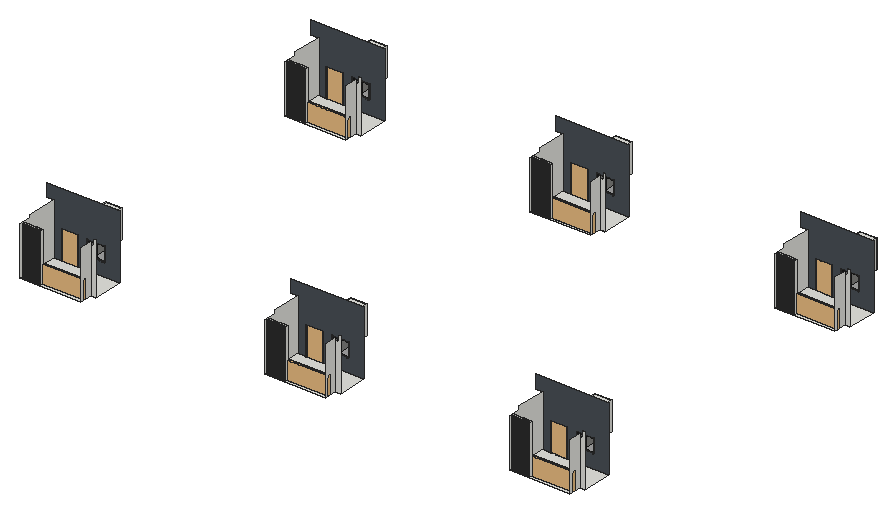
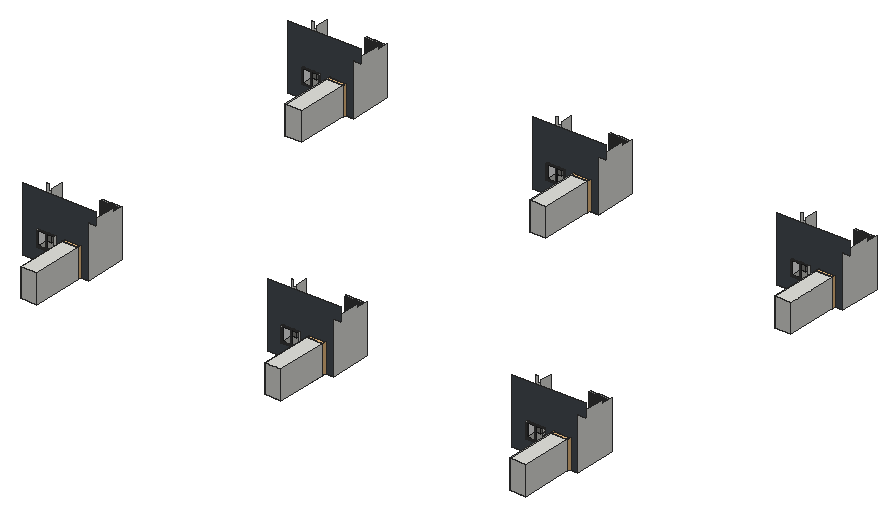
# SketchUp Ruby script. Lengths in inches.
U = 1.inch
M = Sketchup.active_model
def pt(a) = Geom::Point3d.new(a.map { |v| v * U })
def face(e, loops, mat)
  f = e.add_face(loops[0].map { |a| pt(a) })
  loops[1..].each { |l| e.add_face(l.map { |a| pt(a) }).erase! }
  f.material = f.back_material = mat if mat
  f
end
# faces: each face lists its corners as indices into pts; further lists are holes
def faces(e, pts, list, mat = nil) = list.each { |f| face(e, (f[0].is_a?(Array) ? f : [f]).map { |l| l.map { |i| pts[i] } }, mat) }
# xy, xz, yz: faces in a plane at the given z, y or x. An outline is a flat list of corners, or four numbers for a rectangle; further outlines are holes
def ring(l) = l.size == 4 ? [[l[0], l[1]], [l[2], l[1]], [l[2], l[3]], [l[0], l[3]]] : l.each_slice(2).to_a
def flat(e, list, mat, &to3) = list.each { |f| face(e, (f[0].is_a?(Array) ? f : [f]).map { |l| ring(l).map { |u, v| to3.(u, v) } }, mat) }
def xy(e, z, list, mat = nil) = flat(e, list, mat) { |x, y| [x, y, z] }
def xz(e, y, list, mat = nil) = flat(e, list, mat) { |x, z| [x, y, z] }
def yz(e, x, list, mat = nil) = flat(e, list, mat) { |y, z| [x, y, z] }
def lines(e, pts, list) = list.each { |a, b| e.add_line(pt(pts[a]), pt(pts[b])) }
# prism: a flat outline (further loops are holes) pulled along v
def prism(e, loops, v, mat = nil)
  f = face(e, loops, mat); d = Geom::Vector3d.new(v.map { |x| x * U })
  f.pushpull(f.normal.samedirection?(d) ? d.length : -d.length)
end
def box(e, o, s, mat = nil) = prism(e, [[o, [o[0] + s[0], o[1], o[2]], [o[0] + s[0], o[1] + s[1], o[2]], [o[0], o[1] + s[1], o[2]]]], [0, 0, s[2]], mat)
def at(x, y, z, deg = 0) = Geom::Transformation.translation(pt([x, y, z])) * Geom::Transformation.rotation(ORIGIN, Z_AXIS, deg.degrees)
def axes(o, x, y, z) = Geom::Transformation.new([*x, 0, *y, 0, *z, 0, *pt(o).to_a, 1])
def part(name) = M.definitions.add(name)
# library, detail: a bought-in or finely detailed component or shape, given as its bounding box
def library(name, o, s) = part(name).tap { |d| box(d.entities, o, s) }
def detail(e, o, s) = box(e.add_group.entities, o, s)
def put(e, d, t, mat = nil) = e.add_instance(d, t).tap { |i| i.material = mat if mat }
def group(e, t, mat = nil) = e.add_group.tap { |g| g.transformation = t; g.material = mat if mat }.entities
root = M.entities
M.materials.add("Glass_Tinted_Gray").color = [0, 0, 0]
M.materials["Glass_Tinted_Gray"].alpha = 0.125
M.materials.add("[0030_OldLace]").color = [86, 53, 24]
M.materials.add("[0135_DarkGray]").color = [81, 81, 81]
M.materials.add("[Formica Blue]").color = [73, 80, 86]
M.materials.add("[Mirror 02]").color = [229, 229, 229]
M.materials.add("[Terrazzo Light Blue]").color = [196, 214, 227]
c1 = library("Glass Railing",[0,0,0],[139.5,4.76,42])
c2 = library("door (1)",[38.93,25.48,0],[40,9.94,82.68])
c3 = part("PENTEK_RP Fineline 50S_Sliding_DoorCase_E1")
box(c3.entities,[0,0,0],[1.51,3.66,99.27],"[0135_DarkGray]")
c4 = part("PENTEK_RP Fineline 50S_SlidingDooe_Case_E2")
box(c4.entities,[0,0,0],[96.25,3.66,1.51],"[0135_DarkGray]")
c5 = part("pentek_RP Fineline 50S_SlidingDoor_Case")
put(c5.entities,c3,at(97.76,0,0))
put(c5.entities,c4,at(1.51,0,0))
put(c5.entities,c3,at(0,0,0))
put(c5.entities,c4,at(1.51,0,97.76))
c6 = part("PENTEK_RP Fineline 50S_SlidingDoor_GlazingBead_2")
box(c6.entities,[0,0,0],[0.56,0.59,94.39],"[0135_DarkGray]")
c7 = part("PENTEK_RP Fineline 50S_SlidingDoor_Glass")
box(c7.entities,[0,0,0],[46.58,0.16,94.39],"Glass_Tinted_Gray")
c8 = part("PENTEK_RP Fineline 50S_SlidingDoor_GlazingBead")
box(c8.entities,[0,0,0],[45.47,0.59,0.56],"[0135_DarkGray]")
c9 = part("PENTEK_RP Fineline 50S_SlidingDoor_Leaf_E1")
xy(c9.entities,0,[[0,0,0.93,1.97],[0.93,1.57,1.49,1.97]],"[0135_DarkGray]")
xy(c9.entities,96.25,[[0,0,0.93,0,0.93,1.57,1.49,1.57,1.49,1.97,0,1.97]],"[0135_DarkGray]")
xz(c9.entities,0,[[0,0,0.93,96.25]],"[0135_DarkGray]")
xz(c9.entities,1.57,[[0.93,0,1.49,95.32],[0.93,95.32,1.49,96.25]],"[0135_DarkGray]")
xz(c9.entities,1.97,[[0,0,1.49,96.25]],"[0135_DarkGray]")
yz(c9.entities,0,[[0,0,1.97,96.25]],"[0135_DarkGray]")
yz(c9.entities,0.93,[[0,0,1.57,0.93],[0,0.93,1.57,95.32],[0,95.32,1.57,96.25]],"[0135_DarkGray]")
yz(c9.entities,1.49,[[1.57,0,1.97,95.32],[1.57,95.32,1.97,96.25]],"[0135_DarkGray]")
c10 = part("PENTEK_RP Fineline 50S_SlidingDoor_Leaf_E2")
xy(c10.entities,0,[[0,0,0,1.57,0.56,1.57,0.56,1.97,46.02,1.97,46.02,1.57,46.58,1.57,46.58,0]],"[0135_DarkGray]")
xy(c10.entities,0.93,[[0,0,46.58,1.57]],"[0135_DarkGray]")
xy(c10.entities,1.49,[[0.56,1.57,46.02,1.97]],"[0135_DarkGray]")
xz(c10.entities,0,[[0,0,46.58,0.93]],"[0135_DarkGray]")
xz(c10.entities,1.57,[[0,0,0.56,0.93],[46.02,0,46.58,0.93],[0.56,0.93,46.02,1.49]],"[0135_DarkGray]")
xz(c10.entities,1.97,[[0.56,0,46.02,1.49]],"[0135_DarkGray]")
yz(c10.entities,0,[[0,0,1.57,0.93]],"[0135_DarkGray]")
yz(c10.entities,0.56,[[1.57,0,1.97,0.93],[1.57,0.93,1.97,1.49]],"[0135_DarkGray]")
yz(c10.entities,46.02,[[1.57,0,1.97,0.93],[1.57,0.93,1.97,1.49]],"[0135_DarkGray]")
yz(c10.entities,46.58,[[0,0,1.57,0.93]],"[0135_DarkGray]")
c11 = part("PENTEK_RP Fineline S_SlidingDoor_Leaf1")
put(c11.entities,c6,at(0.93,0,0.93))
put(c11.entities,c6,at(46.96,0,0.93))
put(c11.entities,c7,at(1.49,1.42,0.93))
put(c11.entities,c8,at(1.49,0,0.93))
put(c11.entities,c7,at(1.49,0.59,0.93),"[Terrazzo Light Blue]")
put(c11.entities,c9,at(0,0,0))
put(c11.entities,c9,axes([48.44,0,0],[-1,0,0],[0,1,0],[0,0,1]))
put(c11.entities,c10,axes([0.93,0,96.25],[1,0,0],[0,1,0],[0,0,-1]))
put(c11.entities,c10,at(0.93,0,0))
put(c11.entities,c8,at(1.49,0,94.77))
c12 = part("PENTEK_RP Fineline 50S_SlidingDoor_Leaf2")
put(c12.entities,c7,at(1.49,1.42,0.93))
put(c12.entities,c8,at(1.49,0,94.77))
put(c12.entities,c6,at(46.96,0,0.93))
put(c12.entities,c7,at(1.49,0.59,0.93),"[Mirror 02]")
put(c12.entities,c6,at(0.93,0,0.93))
put(c12.entities,c9,at(0,0,0))
put(c12.entities,c9,axes([48.44,0,0],[-1,0,0],[0,1,0],[0,0,1]))
put(c12.entities,c8,at(1.49,0,0.93))
put(c12.entities,c10,axes([0.93,0,96.25],[1,0,0],[0,1,0],[0,0,-1]))
put(c12.entities,c10,at(0.93,0,0))
c13 = part("PENTEK - Slimmest Steel Sliding Door / Window\#1")
put(c13.entities,c5,at(0,-1.88,-0.09))
put(c13.entities,c11,at(1.51,-2.27,1.42))
put(c13.entities,c12,at(49.32,-0.3,1.42))
xy(root,526.75,[[[158.83,412.04,338.6875,412.04,338.6875,447.84,353.97,447.84,353.97,535.375,158.83,535.375],[161.79,416.2,166.6,422.7],[168.1,416.2,172.92,422.7],[174.42,416.2,179.23,422.7],[180.67,416.2,185.48,422.7],[186.92,416.2,191.73,422.7],[193.17,416.2,197.98,422.7],[199.42,416.2,204.23,422.7],[205.67,416.2,210.48,422.7],[211.92,416.2,216.73,422.7]],[[883.27,412.04,1063.125,412.04,1063.125,447.84,1078.41,447.84,1078.41,535.375,883.27,535.375],[886.23,416.2,891.04,422.7],[892.54,416.2,897.35,422.7],[898.85,416.2,903.67,422.7],[905.1,416.2,909.92,422.7],[911.35,416.2,916.17,422.7],[917.6,416.2,922.42,422.7],[923.85,416.2,928.67,422.7],[930.1,416.2,934.92,422.7],[936.35,416.2,941.17,422.7]],[[1607.71,412.04,1787.5625,412.04,1787.5625,447.84,1802.84,447.84,1802.84,535.375,1607.71,535.375],[1610.67,416.2,1615.48,422.7],[1616.98,416.2,1621.79,422.7],[1623.29,416.2,1628.1,422.7],[1629.54,416.2,1634.35,422.7],[1635.79,416.2,1640.6,422.7],[1642.04,416.2,1646.85,422.7],[1648.29,416.2,1653.1,422.7],[1654.54,416.2,1659.35,422.7],[1660.79,416.2,1665.6,422.7]],[183.3,535.375,231.3,699.0625],[907.74,535.375,955.74,699.0625],
  [1632.17,535.375,1680.17,699.0625],[[158.83,1392.39,338.6875,1392.39,338.6875,1428.19,353.97,1428.19,353.97,1515.73,158.83,1515.73],[161.79,1396.55,166.6,1403.05],[168.1,1396.55,172.92,1403.05],[174.42,1396.55,179.23,1403.05],[180.67,1396.55,185.48,1403.05],[186.92,1396.55,191.73,1403.05],[193.17,1396.55,197.98,1403.05],[199.42,1396.55,204.23,1403.05],[205.67,1396.55,210.48,1403.05],[211.92,1396.55,216.73,1403.05]],[[883.27,1392.39,1063.125,1392.39,1063.125,1428.19,1078.41,1428.19,1078.41,1515.73,883.27,1515.73],[886.23,1396.55,891.04,1403.05],[892.54,1396.55,897.35,1403.05],[898.85,1396.55,903.67,1403.05],[905.1,1396.55,909.92,1403.05],[911.35,1396.55,916.17,1403.05],[917.6,1396.55,922.42,1403.05],[923.85,1396.55,928.67,1403.05],[930.1,1396.55,934.92,1403.05],[936.35,1396.55,941.17,1403.05]],[[1607.71,1392.39,1787.5625,1392.39,1787.5625,1428.19,1802.84,1428.19,1802.84,1515.73,1607.71,1515.73],[1610.67,1396.55,1615.48,1403.05],[1616.98,1396.55,1621.79,1403.05],[1623.29,1396.55,1628.1,1403.05],[1629.54,1396.55,1634.35,1403.05],[1635.79,1396.55,1640.6,1403.05],[1642.04,1396.55,1646.85,1403.05],[1648.29,1396.55,1653.1,1403.05],[1654.54,1396.55,1659.35,1403.05],[1660.79,1396.55,1665.6,1403.05]],[183.3,1515.73,231.3,1679.41],
  [907.74,1515.73,955.74,1679.41],[1632.17,1515.73,1680.17,1679.41]])
xy(root,566.5625,[[258.09,535.375,309.84,540.48],[982.53,535.375,1034.28,540.48],[1706.96,535.375,1758.71,540.48],[258.09,1515.73,309.84,1520.83],[982.53,1515.73,1034.28,1520.83],
  [1706.96,1515.73,1758.71,1520.83]])
xy(root,610.75,[[183.3,535.375,231.3,699.0625],[258.09,535.375,309.84,540.48],[907.74,535.375,955.74,699.0625],[982.53,535.375,1034.28,540.48],[1632.17,535.375,1680.17,699.0625],
  [1706.96,535.375,1758.71,540.48],[183.3,1515.73,231.3,1679.41],[258.09,1515.73,309.84,1520.83],[907.74,1515.73,955.74,1679.41],[982.53,1515.73,1034.28,1520.83],
  [1632.17,1515.73,1680.17,1679.41],[1706.96,1515.73,1758.71,1520.83]])
xz(root,416.2,[[161.79,526.75,166.6,669.8125],[168.1,526.75,172.92,669.8125],[174.42,526.75,179.23,669.8125],[180.67,526.75,185.48,669.8125],[186.92,526.75,191.73,669.8125],
  [193.17,526.75,197.98,669.8125],[199.42,526.75,204.23,669.8125],[205.67,526.75,210.48,669.8125],[211.92,526.75,216.73,669.8125],[1610.67,526.75,1615.48,669.8125],
  [1616.98,526.75,1621.79,669.8125],[1623.29,526.75,1628.1,669.8125],[1629.54,526.75,1634.35,669.8125],[1635.79,526.75,1640.6,669.8125],[1642.04,526.75,1646.85,669.8125],
  [1648.29,526.75,1653.1,669.8125],[1654.54,526.75,1659.35,669.8125],[1660.79,526.75,1665.6,669.8125]])
xz(root,416.2,[[886.23,526.75,891.04,669.8125],[892.54,526.75,897.35,669.8125],[898.85,526.75,903.67,669.8125],[905.1,526.75,909.92,669.8125],[911.35,526.75,916.17,669.8125],
  [917.6,526.75,922.42,669.8125],[923.85,526.75,928.67,669.8125],[930.1,526.75,934.92,669.8125],[936.35,526.75,941.17,669.8125]],"[0030_OldLace]")
xz(root,422.7,[[161.79,526.75,166.6,669.8125],[168.1,526.75,172.92,669.8125],[174.42,526.75,179.23,669.8125],[180.67,526.75,185.48,669.8125],[186.92,526.75,191.73,669.8125],
  [193.17,526.75,197.98,669.8125],[199.42,526.75,204.23,669.8125],[205.67,526.75,210.48,669.8125],[211.92,526.75,216.73,669.8125],[886.23,526.75,891.04,669.8125],
  [892.54,526.75,897.35,669.8125],[898.85,526.75,903.67,669.8125],[905.1,526.75,909.92,669.8125],[911.35,526.75,916.17,669.8125],[917.6,526.75,922.42,669.8125],
  [923.85,526.75,928.67,669.8125],[930.1,526.75,934.92,669.8125],[936.35,526.75,941.17,669.8125],[1610.67,526.75,1615.48,669.8125],[1616.98,526.75,1621.79,669.8125],
  [1623.29,526.75,1628.1,669.8125],[1629.54,526.75,1634.35,669.8125],[1635.79,526.75,1640.6,669.8125],[1642.04,526.75,1646.85,669.8125],[1648.29,526.75,1653.1,669.8125],
  [1654.54,526.75,1659.35,669.8125],[1660.79,526.75,1665.6,669.8125]])
xz(root,447.84,[[338.6875,526.75,338.6875,662.8125,348.1875,662.8125,348.1875,679.3125,353.97,679.3125,353.97,526.75],[1063.125,526.75,1063.125,662.8125,1072.625,662.8125,1072.625,679.3125,1078.41,679.3125,1078.41,526.75],[1787.5625,526.75,1787.5625,662.8125,1797.0625,662.8125,1797.0625,679.3125,1802.84,679.3125,1802.84,526.75]])
xz(root,535.375,[[[158.83,526.75,183.3,526.75,183.3,610.75,231.3,610.75,231.3,526.75,353.97,526.75,353.97,718,137.5,718,137.5,679.3125,158.83,679.3125],[258.09,566.5625,309.84,610.75]],[[883.27,526.75,907.74,526.75,907.74,610.75,955.74,610.75,955.74,526.75,1078.41,526.75,1078.41,718,861.9375,718,861.9375,679.3125,883.27,679.3125],[982.53,566.5625,1034.28,610.75]],[[1607.71,526.75,1632.17,526.75,1632.17,610.75,1680.17,610.75,1680.17,526.75,1802.84,526.75,1802.84,718,1586.375,718,1586.375,679.3125,1607.71,679.3125],[1706.96,566.5625,1758.71,610.75]]],"[Formica Blue]")
xz(root,699.0625,[[183.3,526.75,231.3,610.75],[907.74,526.75,955.74,610.75],[1632.17,526.75,1680.17,610.75]])
xz(root,1396.55,[[161.79,526.75,166.6,669.8125],[168.1,526.75,172.92,669.8125],[174.42,526.75,179.23,669.8125],[180.67,526.75,185.48,669.8125],[186.92,526.75,191.73,669.8125],
  [193.17,526.75,197.98,669.8125],[199.42,526.75,204.23,669.8125],[205.67,526.75,210.48,669.8125],[211.92,526.75,216.73,669.8125],[886.23,526.75,891.04,669.8125],
  [892.54,526.75,897.35,669.8125],[898.85,526.75,903.67,669.8125],[905.1,526.75,909.92,669.8125],[911.35,526.75,916.17,669.8125],[917.6,526.75,922.42,669.8125],
  [923.85,526.75,928.67,669.8125],[930.1,526.75,934.92,669.8125],[936.35,526.75,941.17,669.8125],[1610.67,526.75,1615.48,669.8125],[1616.98,526.75,1621.79,669.8125],
  [1623.29,526.75,1628.1,669.8125],[1629.54,526.75,1634.35,669.8125],[1635.79,526.75,1640.6,669.8125],[1642.04,526.75,1646.85,669.8125],[1648.29,526.75,1653.1,669.8125],
  [1654.54,526.75,1659.35,669.8125],[1660.79,526.75,1665.6,669.8125]])
xz(root,1403.05,[[161.79,526.75,166.6,669.8125],[168.1,526.75,172.92,669.8125],[174.42,526.75,179.23,669.8125],[180.67,526.75,185.48,669.8125],[186.92,526.75,191.73,669.8125],
  [193.17,526.75,197.98,669.8125],[199.42,526.75,204.23,669.8125],[205.67,526.75,210.48,669.8125],[211.92,526.75,216.73,669.8125],[886.23,526.75,891.04,669.8125],
  [892.54,526.75,897.35,669.8125],[898.85,526.75,903.67,669.8125],[905.1,526.75,909.92,669.8125],[911.35,526.75,916.17,669.8125],[917.6,526.75,922.42,669.8125],
  [923.85,526.75,928.67,669.8125],[930.1,526.75,934.92,669.8125],[936.35,526.75,941.17,669.8125],[1610.67,526.75,1615.48,669.8125],[1616.98,526.75,1621.79,669.8125],
  [1623.29,526.75,1628.1,669.8125],[1629.54,526.75,1634.35,669.8125],[1635.79,526.75,1640.6,669.8125],[1642.04,526.75,1646.85,669.8125],[1648.29,526.75,1653.1,669.8125],
  [1654.54,526.75,1659.35,669.8125],[1660.79,526.75,1665.6,669.8125]])
xz(root,1428.19,[[338.6875,526.75,338.6875,662.8125,348.1875,662.8125,348.1875,679.3125,353.97,679.3125,353.97,526.75],[1063.125,526.75,1063.125,662.8125,1072.625,662.8125,1072.625,679.3125,1078.41,679.3125,1078.41,526.75],[1787.5625,526.75,1787.5625,662.8125,1797.0625,662.8125,1797.0625,679.3125,1802.84,679.3125,1802.84,526.75]])
xz(root,1515.73,[[[158.83,526.75,183.3,526.75,183.3,610.75,231.3,610.75,231.3,526.75,353.97,526.75,353.97,718,137.5,718,137.5,679.3125,158.83,679.3125],[258.09,566.5625,309.84,610.75]],[[883.27,526.75,907.74,526.75,907.74,610.75,955.74,610.75,955.74,526.75,1078.41,526.75,1078.41,718,861.9375,718,861.9375,679.3125,883.27,679.3125],[982.53,566.5625,1034.28,610.75]],[[1607.71,526.75,1632.17,526.75,1632.17,610.75,1680.17,610.75,1680.17,526.75,1802.84,526.75,1802.84,718,1586.375,718,1586.375,679.3125,1607.71,679.3125],[1706.96,566.5625,1758.71,610.75]]],"[Formica Blue]")
xz(root,1679.41,[[183.3,526.75,231.3,610.75],[907.74,526.75,955.74,610.75],[1632.17,526.75,1680.17,610.75]])
yz(root,158.83,[[412.04,526.75,535.375,526.75,535.375,679.3125,447.84,679.3125,447.84,669.8125,412.04,669.8125],[1392.39,526.75,1515.73,526.75,1515.73,679.3125,1428.19,679.3125,1428.19,669.8125,1392.39,669.8125]])
yz(root,161.79,[[416.2,526.75,422.7,669.8125],[1396.55,526.75,1403.05,669.8125]])
yz(root,166.6,[[416.2,526.75,422.7,669.8125],[1396.55,526.75,1403.05,669.8125]])
yz(root,168.1,[[416.2,526.75,422.7,669.8125],[1396.55,526.75,1403.05,669.8125]])
yz(root,172.92,[[416.2,526.75,422.7,669.8125],[1396.55,526.75,1403.05,669.8125]])
yz(root,174.42,[[416.2,526.75,422.7,669.8125],[1396.55,526.75,1403.05,669.8125]])
yz(root,179.23,[[416.2,526.75,422.7,669.8125],[1396.55,526.75,1403.05,669.8125]])
yz(root,180.67,[[416.2,526.75,422.7,669.8125],[1396.55,526.75,1403.05,669.8125]])
yz(root,183.3,[[535.375,526.75,699.0625,610.75],[1515.73,526.75,1679.41,610.75]])
yz(root,185.48,[[416.2,526.75,422.7,669.8125],[1396.55,526.75,1403.05,669.8125]])
yz(root,186.92,[[416.2,526.75,422.7,669.8125],[1396.55,526.75,1403.05,669.8125]])
yz(root,191.73,[[416.2,526.75,422.7,669.8125],[1396.55,526.75,1403.05,669.8125]])
yz(root,193.17,[[416.2,526.75,422.7,669.8125],[1396.55,526.75,1403.05,669.8125]])
yz(root,197.98,[[416.2,526.75,422.7,669.8125],[1396.55,526.75,1403.05,669.8125]])
yz(root,199.42,[[416.2,526.75,422.7,669.8125],[1396.55,526.75,1403.05,669.8125]])
yz(root,204.23,[[416.2,526.75,422.7,669.8125],[1396.55,526.75,1403.05,669.8125]])
yz(root,205.67,[[416.2,526.75,422.7,669.8125],[1396.55,526.75,1403.05,669.8125]])
yz(root,210.48,[[416.2,526.75,422.7,669.8125],[1396.55,526.75,1403.05,669.8125]])
yz(root,211.92,[[416.2,526.75,422.7,669.8125],[1396.55,526.75,1403.05,669.8125]])
yz(root,216.73,[[416.2,526.75,422.7,669.8125],[1396.55,526.75,1403.05,669.8125]])
yz(root,231.3,[[535.375,526.75,699.0625,610.75],[1515.73,526.75,1679.41,610.75]])
yz(root,258.09,[[535.375,566.5625,540.48,610.75],[1515.73,566.5625,1520.83,610.75]])
yz(root,309.84,[[535.375,566.5625,540.48,610.75],[1515.73,566.5625,1520.83,610.75]])
yz(root,338.6875,[[412.04,526.75,447.84,669.8125],[1392.39,526.75,1428.19,669.8125]])
yz(root,883.27,[[412.04,526.75,535.375,526.75,535.375,679.3125,447.84,679.3125,447.84,669.8125,412.04,669.8125],[1392.39,526.75,1515.73,526.75,1515.73,679.3125,1428.19,679.3125,1428.19,669.8125,1392.39,669.8125]])
yz(root,886.23,[[416.2,526.75,422.7,669.8125],[1396.55,526.75,1403.05,669.8125]])
yz(root,891.04,[[416.2,526.75,422.7,669.8125],[1396.55,526.75,1403.05,669.8125]])
yz(root,892.54,[[416.2,526.75,422.7,669.8125],[1396.55,526.75,1403.05,669.8125]])
yz(root,897.35,[[416.2,526.75,422.7,669.8125],[1396.55,526.75,1403.05,669.8125]])
yz(root,898.85,[[416.2,526.75,422.7,669.8125],[1396.55,526.75,1403.05,669.8125]])
yz(root,903.67,[[416.2,526.75,422.7,669.8125],[1396.55,526.75,1403.05,669.8125]])
yz(root,905.1,[[416.2,526.75,422.7,669.8125],[1396.55,526.75,1403.05,669.8125]])
yz(root,907.74,[[535.375,526.75,699.0625,610.75],[1515.73,526.75,1679.41,610.75]])
yz(root,909.92,[[416.2,526.75,422.7,669.8125],[1396.55,526.75,1403.05,669.8125]])
yz(root,911.35,[[416.2,526.75,422.7,669.8125],[1396.55,526.75,1403.05,669.8125]])
yz(root,916.17,[[416.2,526.75,422.7,669.8125],[1396.55,526.75,1403.05,669.8125]])
yz(root,917.6,[[416.2,526.75,422.7,669.8125],[1396.55,526.75,1403.05,669.8125]])
yz(root,922.42,[[416.2,526.75,422.7,669.8125],[1396.55,526.75,1403.05,669.8125]])
yz(root,923.85,[[416.2,526.75,422.7,669.8125],[1396.55,526.75,1403.05,669.8125]])
yz(root,928.67,[[416.2,526.75,422.7,669.8125],[1396.55,526.75,1403.05,669.8125]])
yz(root,930.1,[[416.2,526.75,422.7,669.8125],[1396.55,526.75,1403.05,669.8125]])
yz(root,934.92,[[416.2,526.75,422.7,669.8125],[1396.55,526.75,1403.05,669.8125]])
yz(root,936.35,[[416.2,526.75,422.7,669.8125],[1396.55,526.75,1403.05,669.8125]])
yz(root,941.17,[[416.2,526.75,422.7,669.8125],[1396.55,526.75,1403.05,669.8125]])
yz(root,955.74,[[535.375,526.75,699.0625,610.75],[1515.73,526.75,1679.41,610.75]])
yz(root,982.53,[[535.375,566.5625,540.48,610.75],[1515.73,566.5625,1520.83,610.75]])
yz(root,1034.28,[[535.375,566.5625,540.48,610.75],[1515.73,566.5625,1520.83,610.75]])
yz(root,1063.125,[[412.04,526.75,447.84,669.8125],[1392.39,526.75,1428.19,669.8125]])
yz(root,1607.71,[[412.04,526.75,535.375,526.75,535.375,679.3125,447.84,679.3125,447.84,669.8125,412.04,669.8125],[1392.39,526.75,1515.73,526.75,1515.73,679.3125,1428.19,679.3125,1428.19,669.8125,1392.39,669.8125]])
yz(root,1610.67,[[416.2,526.75,422.7,669.8125],[1396.55,526.75,1403.05,669.8125]])
yz(root,1615.48,[[416.2,526.75,422.7,669.8125],[1396.55,526.75,1403.05,669.8125]])
yz(root,1616.98,[[416.2,526.75,422.7,669.8125],[1396.55,526.75,1403.05,669.8125]])
yz(root,1621.79,[[416.2,526.75,422.7,669.8125],[1396.55,526.75,1403.05,669.8125]])
yz(root,1623.29,[[416.2,526.75,422.7,669.8125],[1396.55,526.75,1403.05,669.8125]])
yz(root,1628.1,[[416.2,526.75,422.7,669.8125],[1396.55,526.75,1403.05,669.8125]])
yz(root,1629.54,[[416.2,526.75,422.7,669.8125],[1396.55,526.75,1403.05,669.8125]])
yz(root,1632.17,[[535.375,526.75,699.0625,610.75],[1515.73,526.75,1679.41,610.75]])
yz(root,1634.35,[[416.2,526.75,422.7,669.8125],[1396.55,526.75,1403.05,669.8125]])
yz(root,1635.79,[[416.2,526.75,422.7,669.8125],[1396.55,526.75,1403.05,669.8125]])
yz(root,1640.6,[[416.2,526.75,422.7,669.8125],[1396.55,526.75,1403.05,669.8125]])
yz(root,1642.04,[[416.2,526.75,422.7,669.8125],[1396.55,526.75,1403.05,669.8125]])
yz(root,1646.85,[[416.2,526.75,422.7,669.8125],[1396.55,526.75,1403.05,669.8125]])
yz(root,1648.29,[[416.2,526.75,422.7,669.8125],[1396.55,526.75,1403.05,669.8125]])
yz(root,1653.1,[[416.2,526.75,422.7,669.8125],[1396.55,526.75,1403.05,669.8125]])
yz(root,1654.54,[[416.2,526.75,422.7,669.8125],[1396.55,526.75,1403.05,669.8125]])
yz(root,1659.35,[[416.2,526.75,422.7,669.8125],[1396.55,526.75,1403.05,669.8125]])
yz(root,1660.79,[[416.2,526.75,422.7,669.8125],[1396.55,526.75,1403.05,669.8125]])
yz(root,1665.6,[[416.2,526.75,422.7,669.8125],[1396.55,526.75,1403.05,669.8125]])
yz(root,1680.17,[[535.375,526.75,699.0625,610.75],[1515.73,526.75,1679.41,610.75]])
yz(root,1706.96,[[535.375,566.5625,540.48,610.75],[1515.73,566.5625,1520.83,610.75]])
yz(root,1758.71,[[535.375,566.5625,540.48,610.75],[1515.73,566.5625,1520.83,610.75]])
yz(root,1787.5625,[[412.04,526.75,447.84,669.8125],[1392.39,526.75,1428.19,669.8125]])
put(root,c1,axes([161.79,1401.14,526.75],[1.27,0,0],[0,1.27,0],[0,0,1.27]))
put(root,c1,axes([886.23,1401.14,526.75],[1.27,0,0],[0,1.27,0],[0,0,1.27]))
put(root,c1,axes([1610.67,1401.14,526.75],[1.27,0,0],[0,1.27,0],[0,0,1.27]))
put(root,c1,axes([886.23,420.79,526.75],[1.27,0,0],[0,1.27,0],[0,0,1.27]))
put(root,c1,axes([1610.67,420.79,526.75],[1.27,0,0],[0,1.27,0],[0,0,1.27]))
put(root,c1,axes([161.79,420.79,526.75],[1.27,0,0],[0,1.27,0],[0,0,1.27]))
put(root,c2,axes([1582.69,1490.24,526.75],[1.2351,0,0],[0,1,0],[0,0,1.016]))
put(root,c2,axes([133.81,1490.24,526.75],[1.2351,0,0],[0,1,0],[0,0,1.016]))
put(root,c2,axes([858.25,1490.24,526.75],[1.2351,0,0],[0,1,0],[0,0,1.016]))
put(root,c2,axes([858.25,509.89,526.75],[1.2351,0,0],[0,1,0],[0,0,1.016]))
put(root,c2,axes([1582.69,509.89,526.75],[1.2351,0,0],[0,1,0],[0,0,1.016]))
put(root,c2,axes([133.81,509.89,526.75],[1.2351,0,0],[0,1,0],[0,0,1.016]))
put(root,c13,axes([258.09,1516.73,566.51],[0.52129,0,0],[0,0.44,0],[0,0,0.44603]))
put(root,c13,axes([1706.96,1516.73,566.51],[0.52129,0,0],[0,0.44,0],[0,0,0.44603]))
put(root,c13,axes([982.53,1516.73,566.51],[0.52129,0,0],[0,0.44,0],[0,0,0.44603]))
put(root,c13,axes([982.53,536.375,566.51],[0.52129,0,0],[0,0.44,0],[0,0,0.44603]))
put(root,c13,axes([1706.96,536.375,566.51],[0.52129,0,0],[0,0.44,0],[0,0,0.44603]))
put(root,c13,axes([258.09,536.375,566.51],[0.52129,0,0],[0,0.44,0],[0,0,0.44603]))
